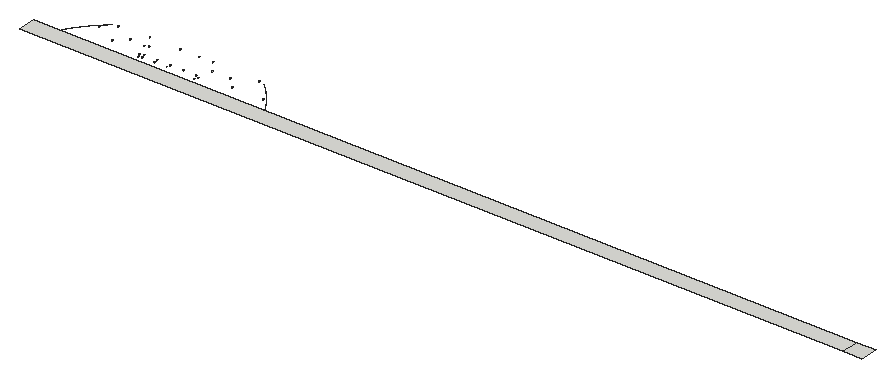
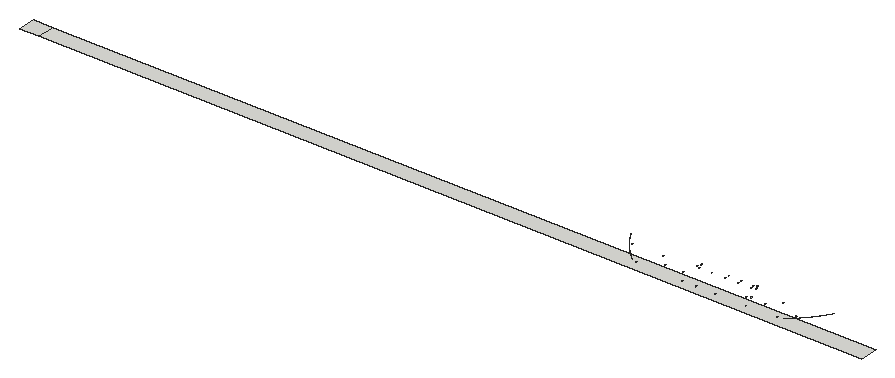
# SketchUp Ruby script. Lengths in inches.
U = 1.inch
M = Sketchup.active_model
def pt(a) = Geom::Point3d.new(a.map { |v| v * U })
def face(e, loops, mat)
  f = e.add_face(loops[0].map { |a| pt(a) })
  loops[1..].each { |l| e.add_face(l.map { |a| pt(a) }).erase! }
  f.material = f.back_material = mat if mat
  f
end
# faces: each face lists its corners as indices into pts; further lists are holes
def faces(e, pts, list, mat = nil) = list.each { |f| face(e, (f[0].is_a?(Array) ? f : [f]).map { |l| l.map { |i| pts[i] } }, mat) }
# xy, xz, yz: faces in a plane at the given z, y or x. An outline is a flat list of corners, or four numbers for a rectangle; further outlines are holes
def ring(l) = l.size == 4 ? [[l[0], l[1]], [l[2], l[1]], [l[2], l[3]], [l[0], l[3]]] : l.each_slice(2).to_a
def flat(e, list, mat, &to3) = list.each { |f| face(e, (f[0].is_a?(Array) ? f : [f]).map { |l| ring(l).map { |u, v| to3.(u, v) } }, mat) }
def xy(e, z, list, mat = nil) = flat(e, list, mat) { |x, y| [x, y, z] }
def xz(e, y, list, mat = nil) = flat(e, list, mat) { |x, z| [x, y, z] }
def yz(e, x, list, mat = nil) = flat(e, list, mat) { |y, z| [x, y, z] }
def lines(e, pts, list) = list.each { |a, b| e.add_line(pt(pts[a]), pt(pts[b])) }
# prism: a flat outline (further loops are holes) pulled along v
def prism(e, loops, v, mat = nil)
  f = face(e, loops, mat); d = Geom::Vector3d.new(v.map { |x| x * U })
  f.pushpull(f.normal.samedirection?(d) ? d.length : -d.length)
end
def box(e, o, s, mat = nil) = prism(e, [[o, [o[0] + s[0], o[1], o[2]], [o[0] + s[0], o[1] + s[1], o[2]], [o[0], o[1] + s[1], o[2]]]], [0, 0, s[2]], mat)
def at(x, y, z, deg = 0) = Geom::Transformation.translation(pt([x, y, z])) * Geom::Transformation.rotation(ORIGIN, Z_AXIS, deg.degrees)
def axes(o, x, y, z) = Geom::Transformation.new([*x, 0, *y, 0, *z, 0, *pt(o).to_a, 1])
def part(name) = M.definitions.add(name)
# library, detail: a bought-in or finely detailed component or shape, given as its bounding box
def library(name, o, s) = part(name).tap { |d| box(d.entities, o, s) }
def detail(e, o, s) = box(e.add_group.entities, o, s)
def put(e, d, t, mat = nil) = e.add_instance(d, t).tap { |i| i.material = mat if mat }
def group(e, t, mat = nil) = e.add_group.tap { |g| g.transformation = t; g.material = mat if mat }.entities
root = M.entities
M.materials.add("[Asphalt_Stamped_Brick]").color = [149, 133, 134]
M.materials.add("[Metal_Steel_Textured_White]").color = [191, 191, 191]
xy(root,0,[[116.615,177.536,303.95,181.5],[303.95,177.536,308.325,181.5]])
xy(root,3.625,[[143.477,177.623,143.471,177.624,143.467,177.626,143.463,177.629,143.459,177.633,143.457,177.638,143.457,177.649,143.459,177.653,143.467,177.661,143.471,177.663,143.482,177.663,143.487,177.661,143.491,177.657,143.494,177.653,143.496,177.649,143.497,177.643,143.496,177.638,143.494,177.633,143.491,177.629,143.487,177.626,143.482,177.624],[156.159,177.623,156.154,177.624,156.149,177.626,156.145,177.629,156.142,177.633,156.14,177.638,156.139,177.643,156.14,177.649,156.142,177.653,156.145,177.657,156.149,177.661,156.154,177.663,156.164,177.663,156.169,177.661,156.173,177.657,156.176,177.653,156.178,177.649,156.179,177.643,156.178,177.638,156.176,177.633,156.173,177.629,156.169,177.626,156.164,177.624],[144.214,177.929,144.209,177.93,144.204,177.932,144.2,177.935,144.197,177.939,144.195,177.944,144.194,177.949,144.195,177.954,144.197,177.959,144.2,177.963,144.204,177.966,144.209,177.968,144.214,177.969,144.219,177.968,144.224,177.966,144.228,177.963,144.232,177.959,144.234,177.954,144.234,177.944,144.232,177.939,144.228,177.935,144.224,177.932,144.219,177.93],[147.016,177.929,147.011,177.93,147.006,177.932,147.002,177.935,146.999,177.939,146.997,177.944,146.996,177.949,146.997,177.954,146.999,177.959,147.002,177.963,147.006,177.966,147.011,177.968,147.016,177.969,147.021,177.968,147.026,177.966,147.03,177.963,147.033,177.959,147.035,177.954,147.036,177.949,147.035,177.944,147.033,177.939,147.03,177.935,147.026,177.932,147.021,177.93],[143.141,178.422,143.136,178.424,143.132,178.428,143.129,178.432,143.127,178.437,143.126,178.442,143.127,178.447,143.129,178.452,143.132,178.456,143.136,178.459,143.141,178.461,143.146,178.462,143.151,178.461,143.156,178.459,143.16,178.456,143.163,178.452,143.165,178.447,143.166,178.442,143.165,178.437,143.163,178.432,143.16,178.428,143.156,178.424,143.151,178.422],
  [156.485,178.422,156.48,178.424,156.476,178.428,156.473,178.432,156.471,178.437,156.47,178.442,156.471,178.447,156.473,178.452,156.476,178.456,156.48,178.459,156.485,178.461,156.49,178.462,156.495,178.461,156.5,178.459,156.504,178.456,156.507,178.452,156.509,178.447,156.51,178.442,156.509,178.437,156.507,178.432,156.504,178.428,156.5,178.424,156.495,178.422],[146.851,178.727,146.846,178.728,146.841,178.73,146.837,178.733,146.833,178.737,146.831,178.742,146.831,178.752,146.833,178.757,146.841,178.765,146.846,178.767,146.856,178.767,146.861,178.765,146.865,178.761,146.868,178.757,146.87,178.752,146.871,178.747,146.87,178.742,146.868,178.737,146.865,178.733,146.861,178.73,146.856,178.728],[155.752,178.727,155.747,178.728,155.742,178.73,155.738,178.733,155.735,178.737,155.733,178.742,155.732,178.747,155.733,178.752,155.735,178.757,155.738,178.761,155.742,178.765,155.747,178.767,155.757,178.767,155.762,178.765,155.766,178.761,155.769,178.757,155.771,178.752,155.772,178.747,155.771,178.742,155.769,178.737,155.766,178.733,155.762,178.73,155.757,178.728],[136.121,179.395,136.116,179.396,136.111,179.398,136.107,179.401,136.104,179.405,136.102,179.41,136.101,179.415,136.102,179.42,136.104,179.425,136.107,179.429,136.111,179.433,136.116,179.435,136.126,179.435,136.131,179.433,136.135,179.429,136.138,179.425,136.14,179.42,136.141,179.415,136.14,179.41,136.138,179.405,136.135,179.401,136.131,179.398,136.126,179.396],[163.515,179.395,163.509,179.396,163.505,179.398,163.501,179.401,163.497,179.405,163.495,179.41,163.495,179.42,163.497,179.425,163.505,179.433,163.509,179.435,163.52,179.435,163.525,179.433,163.529,179.429,163.532,179.425,163.534,179.42,163.535,179.415,163.534,179.41,163.532,179.405,163.529,179.401,163.525,179.398,163.52,179.396],
  [142.641,181.727,142.636,181.728,142.631,181.73,142.627,181.733,142.624,181.737,142.622,181.742,142.621,181.747,142.622,181.752,142.624,181.757,142.627,181.761,142.631,181.765,142.636,181.767,142.646,181.767,142.651,181.765,142.655,181.761,142.658,181.757,142.66,181.752,142.661,181.747,142.66,181.742,142.658,181.737,142.655,181.733,142.651,181.73,142.646,181.728],[156.995,181.727,156.99,181.728,156.985,181.73,156.981,181.733,156.978,181.737,156.976,181.742,156.975,181.747,156.976,181.752,156.978,181.757,156.981,181.761,156.985,181.765,156.99,181.767,157,181.767,157.005,181.765,157.009,181.761,157.012,181.757,157.014,181.752,157.015,181.747,157.014,181.742,157.012,181.737,157.009,181.733,157.005,181.73,157,181.728],[161.174,181.736,161.168,181.737,161.164,181.739,161.159,181.742,161.156,181.746,161.154,181.751,161.154,181.761,161.156,181.766,161.159,181.77,161.164,181.774,161.168,181.776,161.179,181.776,161.184,181.774,161.191,181.766,161.193,181.761,161.194,181.756,161.193,181.751,161.191,181.746,161.1875,181.742,161.184,181.739,161.179,181.737],[133.754,184.074,133.748,184.075,133.744,184.077,133.74,184.08,133.736,184.084,133.734,184.089,133.734,184.099,133.736,184.104,133.74,184.108,133.744,184.111,133.748,184.113,133.754,184.114,133.759,184.113,133.764,184.111,133.768,184.108,133.771,184.104,133.773,184.099,133.774,184.094,133.773,184.089,133.771,184.084,133.768,184.08,133.764,184.077,133.759,184.075],[165.882,184.074,165.877,184.075,165.872,184.077,165.868,184.08,165.865,184.084,165.863,184.089,165.862,184.094,165.863,184.099,165.865,184.104,165.868,184.108,165.872,184.111,165.877,184.113,165.882,184.114,165.887,184.113,165.892,184.111,165.896,184.108,165.899,184.104,165.901,184.099,165.902,184.094,165.901,184.089,165.899,184.084,165.896,184.08,165.892,184.077,165.887,184.075],
  [147.578,184.383,147.572,184.384,147.568,184.386,147.564,184.389,147.56,184.393,147.558,184.398,147.558,184.408,147.56,184.413,147.564,184.417,147.568,184.42,147.572,184.422,147.578,184.423,147.583,184.422,147.588,184.42,147.592,184.417,147.595,184.413,147.597,184.408,147.598,184.403,147.597,184.398,147.595,184.393,147.592,184.389,147.588,184.386,147.583,184.384],[155.076,184.383,155.071,184.384,155.066,184.386,155.0625,184.389,155.059,184.393,155.057,184.398,155.057,184.408,155.059,184.413,155.0625,184.417,155.066,184.42,155.071,184.422,155.076,184.423,155.082,184.422,155.086,184.42,155.091,184.417,155.094,184.413,155.096,184.408,155.096,184.398,155.094,184.393,155.091,184.389,155.086,184.386,155.082,184.384],[140.656,184.422,140.651,184.424,140.643,184.432,140.641,184.437,140.641,184.447,140.643,184.452,140.647,184.456,140.651,184.459,140.656,184.461,140.661,184.462,140.666,184.461,140.671,184.459,140.675,184.456,140.678,184.452,140.68,184.447,140.681,184.442,140.68,184.437,140.678,184.432,140.675,184.428,140.671,184.424,140.666,184.422]],"[Asphalt_Stamped_Brick]")
xy(root,3.625,[[[143.477,177.554,143.454,177.557,143.432,177.566,143.414,177.58,143.4,177.599,143.391,177.62,143.388,177.643,143.391,177.666,143.4,177.688,143.414,177.706,143.432,177.72,143.454,177.729,143.477,177.732,143.5,177.729,143.521,177.72,143.539,177.706,143.554,177.688,143.5625,177.666,143.566,177.643,143.5625,177.62,143.554,177.599,143.539,177.58,143.521,177.566,143.5,177.557],[143.477,177.555,143.499,177.558,143.521,177.567,143.539,177.581,143.553,177.599,143.562,177.621,143.565,177.643,143.562,177.666,143.553,177.6875,143.539,177.706,143.521,177.719,143.499,177.728,143.477,177.731,143.454,177.728,143.433,177.719,143.414,177.706,143.401,177.6875,143.392,177.666,143.389,177.643,143.392,177.621,143.401,177.599,143.414,177.581,143.433,177.567,143.454,177.558]],[[156.159,177.554,156.136,177.557,156.115,177.566,156.096,177.58,156.082,177.599,156.073,177.62,156.07,177.643,156.073,177.666,156.082,177.688,156.096,177.706,156.115,177.72,156.136,177.729,156.159,177.732,156.182,177.729,156.204,177.72,156.222,177.706,156.236,177.688,156.245,177.666,156.248,177.643,156.245,177.62,156.236,177.599,156.222,177.58,156.204,177.566,156.182,177.557],[156.159,177.555,156.182,177.558,156.203,177.567,156.221,177.581,156.235,177.599,156.244,177.621,156.247,177.643,156.244,177.666,156.235,177.6875,156.221,177.706,156.203,177.719,156.182,177.728,156.159,177.731,156.136,177.728,156.115,177.719,156.097,177.706,156.083,177.6875,156.074,177.666,156.071,177.643,156.074,177.621,156.083,177.599,156.097,177.581,156.115,177.567,156.136,177.558]],[[143.477,177.555,143.454,177.558,143.433,177.567,143.414,177.581,143.401,177.599,143.392,177.621,143.389,177.643,143.392,177.666,143.401,177.6875,143.414,177.706,143.433,177.719,143.454,177.728,143.477,177.731,143.499,177.728,143.521,177.719,143.539,177.706,143.553,177.6875,143.562,177.666,143.565,177.643,143.562,177.621,143.553,177.599,143.539,177.581,143.521,177.567,143.499,177.558],[143.477,177.607,143.486,177.608,143.495,177.612,143.503,177.617,143.508,177.625,143.512,177.634,143.513,177.643,143.512,177.653,143.508,177.662,143.503,177.669,143.495,177.675,143.486,177.679,143.477,177.68,143.467,177.679,143.458,177.675,143.451,177.669,143.445,177.662,143.441,177.653,143.44,177.643,143.441,177.634,143.445,177.625,143.451,177.617,143.458,177.612,143.467,177.608]],[[156.159,177.555,156.136,177.558,156.115,177.567,156.097,177.581,156.083,177.599,156.074,177.621,156.071,177.643,156.074,177.666,156.083,177.6875,156.097,177.706,156.115,177.719,156.136,177.728,156.159,177.731,156.182,177.728,156.203,177.719,156.221,177.706,156.235,177.6875,156.244,177.666,156.247,177.643,156.244,177.621,156.235,177.599,156.221,177.581,156.203,177.567,156.182,177.558],[156.159,177.607,156.169,177.608,156.177,177.612,156.185,177.617,156.191,177.625,156.194,177.634,156.196,177.643,156.194,177.653,156.191,177.662,156.185,177.669,156.177,177.675,156.169,177.679,156.159,177.68,156.15,177.679,156.141,177.675,156.133,177.669,156.127,177.662,156.124,177.653,156.123,177.643,156.124,177.634,156.127,177.625,156.133,177.617,156.141,177.612,156.15,177.608]],[[143.477,177.607,143.467,177.608,143.458,177.612,143.451,177.617,143.445,177.625,143.441,177.634,143.44,177.643,143.441,177.653,143.445,177.662,143.451,177.669,143.458,177.675,143.467,177.679,143.477,177.68,143.486,177.679,143.495,177.675,143.503,177.669,143.508,177.662,143.512,177.653,143.513,177.643,143.512,177.634,143.508,177.625,143.503,177.617,143.495,177.612,143.486,177.608],[143.477,177.623,143.482,177.624,143.487,177.626,143.491,177.629,143.494,177.633,143.496,177.638,143.497,177.643,143.496,177.649,143.494,177.653,143.491,177.657,143.487,177.661,143.482,177.663,143.471,177.663,143.467,177.661,143.459,177.653,143.457,177.649,143.457,177.638,143.459,177.633,143.463,177.629,143.467,177.626,143.471,177.624]],
  [[144.214,177.861,144.192,177.864,144.17,177.873,144.152,177.887,144.138,177.905,144.129,177.926,144.126,177.949,144.129,177.972,144.138,177.993,144.152,178.011,144.17,178.025,144.192,178.034,144.214,178.037,144.237,178.034,144.258,178.025,144.276,178.011,144.29,177.993,144.299,177.972,144.302,177.949,144.299,177.926,144.29,177.905,144.276,177.887,144.258,177.873,144.237,177.864],[144.214,177.912,144.224,177.914,144.233,177.917,144.24,177.923,144.246,177.931,144.25,177.939,144.251,177.949,144.25,177.958,144.246,177.967,144.24,177.975,144.233,177.981,144.224,177.984,144.214,177.985,144.205,177.984,144.196,177.981,144.188,177.975,144.183,177.967,144.179,177.958,144.178,177.949,144.179,177.939,144.183,177.931,144.188,177.923,144.196,177.917,144.205,177.914]],[[147.016,177.861,146.993,177.864,146.972,177.873,146.954,177.887,146.94,177.905,146.931,177.926,146.928,177.949,146.931,177.972,146.94,177.993,146.954,178.011,146.972,178.025,146.993,178.034,147.016,178.037,147.039,178.034,147.06,178.025,147.078,178.011,147.092,177.993,147.101,177.972,147.104,177.949,147.101,177.926,147.092,177.905,147.078,177.887,147.06,177.873,147.039,177.864],[147.016,177.912,147.026,177.914,147.034,177.917,147.042,177.923,147.048,177.931,147.051,177.939,147.053,177.949,147.051,177.958,147.048,177.967,147.042,177.975,147.034,177.981,147.026,177.984,147.016,177.985,147.007,177.984,146.998,177.981,146.99,177.975,146.984,177.967,146.981,177.958,146.98,177.949,146.981,177.939,146.984,177.931,146.99,177.923,146.998,177.917,147.007,177.914]],[[144.214,177.912,144.205,177.914,144.196,177.917,144.188,177.923,144.183,177.931,144.179,177.939,144.178,177.949,144.179,177.958,144.183,177.967,144.188,177.975,144.196,177.981,144.205,177.984,144.214,177.985,144.224,177.984,144.233,177.981,144.24,177.975,144.246,177.967,144.25,177.958,144.251,177.949,144.25,177.939,144.246,177.931,144.24,177.923,144.233,177.917,144.224,177.914],[144.214,177.929,144.219,177.93,144.224,177.932,144.228,177.935,144.232,177.939,144.234,177.944,144.234,177.954,144.232,177.959,144.228,177.963,144.224,177.966,144.219,177.968,144.214,177.969,144.209,177.968,144.204,177.966,144.2,177.963,144.197,177.959,144.195,177.954,144.194,177.949,144.195,177.944,144.197,177.939,144.2,177.935,144.204,177.932,144.209,177.93]],[[147.016,177.912,147.007,177.914,146.998,177.917,146.99,177.923,146.984,177.931,146.981,177.939,146.98,177.949,146.981,177.958,146.984,177.967,146.99,177.975,146.998,177.981,147.007,177.984,147.016,177.985,147.026,177.984,147.034,177.981,147.042,177.975,147.048,177.967,147.051,177.958,147.053,177.949,147.051,177.939,147.048,177.931,147.042,177.923,147.034,177.917,147.026,177.914],[147.016,177.929,147.021,177.93,147.026,177.932,147.03,177.935,147.033,177.939,147.035,177.944,147.036,177.949,147.035,177.954,147.033,177.959,147.03,177.963,147.026,177.966,147.021,177.968,147.016,177.969,147.011,177.968,147.006,177.966,147.002,177.963,146.999,177.959,146.997,177.954,146.996,177.949,146.997,177.944,146.999,177.939,147.002,177.935,147.006,177.932,147.011,177.93]],[149.818,177.929,149.813,177.93,149.808,177.932,149.804,177.935,149.801,177.939,149.799,177.944,149.798,177.949,149.799,177.954,149.801,177.959,149.804,177.963,149.808,177.966,149.813,177.968,149.818,177.969],
  [149.818,177.929,149.818,177.969,149.823,177.968,149.828,177.966,149.832,177.963,149.835,177.959,149.837,177.954,149.838,177.949,149.837,177.944,149.835,177.939,149.832,177.935,149.828,177.932,149.823,177.93],[[143.146,178.353,143.123,178.356,143.101,178.365,143.083,178.379,143.069,178.397,143.06,178.419,143.057,178.442,143.06,178.465,143.069,178.486,143.083,178.505,143.101,178.519,143.123,178.528,143.146,178.531,143.169,178.528,143.19,178.519,143.209,178.505,143.223,178.486,143.232,178.465,143.235,178.442,143.232,178.419,143.223,178.397,143.209,178.379,143.19,178.365,143.169,178.356],[143.146,178.354,143.169,178.357,143.19,178.366,143.208,178.38,143.222,178.398,143.231,178.419,143.234,178.442,143.231,178.465,143.222,178.486,143.208,178.504,143.19,178.518,143.169,178.527,143.146,178.53,143.123,178.527,143.102,178.518,143.084,178.504,143.07,178.486,143.061,178.465,143.058,178.442,143.061,178.419,143.07,178.398,143.084,178.38,143.102,178.366,143.123,178.357]],[[143.146,178.354,143.123,178.357,143.102,178.366,143.084,178.38,143.07,178.398,143.061,178.419,143.058,178.442,143.061,178.465,143.07,178.486,143.084,178.504,143.102,178.518,143.123,178.527,143.146,178.53,143.169,178.527,143.19,178.518,143.208,178.504,143.222,178.486,143.231,178.465,143.234,178.442,143.231,178.419,143.222,178.398,143.208,178.38,143.19,178.366,143.169,178.357],[143.146,178.405,143.155,178.406,143.164,178.41,143.172,178.416,143.178,178.423,143.181,178.432,143.183,178.442,143.181,178.451,143.178,178.46,143.172,178.468,143.164,178.473,143.155,178.477,143.146,178.478,143.136,178.477,143.128,178.473,143.12,178.468,143.114,178.46,143.111,178.451,143.109,178.442,143.111,178.432,143.114,178.423,143.12,178.416,143.128,178.41,143.136,178.406]],[[143.146,178.405,143.136,178.406,143.128,178.41,143.12,178.416,143.114,178.423,143.111,178.432,143.109,178.442,143.111,178.451,143.114,178.46,143.12,178.468,143.128,178.473,143.136,178.477,143.146,178.478,143.155,178.477,143.164,178.473,143.172,178.468,143.178,178.46,143.181,178.451,143.183,178.442,143.181,178.432,143.178,178.423,143.172,178.416,143.164,178.41,143.155,178.406],[143.141,178.422,143.151,178.422,143.156,178.424,143.16,178.428,143.163,178.432,143.165,178.437,143.166,178.442,143.165,178.447,143.163,178.452,143.16,178.456,143.156,178.459,143.151,178.461,143.146,178.462,143.141,178.461,143.136,178.459,143.132,178.456,143.129,178.452,143.127,178.447,143.126,178.442,143.127,178.437,143.129,178.432,143.132,178.428,143.136,178.424]],[[156.49,178.405,156.48,178.406,156.472,178.41,156.464,178.416,156.458,178.423,156.455,178.432,156.453,178.442,156.455,178.451,156.458,178.46,156.464,178.468,156.472,178.473,156.48,178.477,156.49,178.478,156.499,178.477,156.508,178.473,156.516,178.468,156.522,178.46,156.525,178.451,156.526,178.442,156.525,178.432,156.522,178.423,156.516,178.416,156.508,178.41,156.499,178.406],[156.485,178.422,156.495,178.422,156.5,178.424,156.504,178.428,156.507,178.432,156.509,178.437,156.51,178.442,156.509,178.447,156.507,178.452,156.504,178.456,156.5,178.459,156.495,178.461,156.49,178.462,156.485,178.461,156.48,178.459,156.476,178.456,156.473,178.452,156.471,178.447,156.47,178.442,156.471,178.437,156.473,178.432,156.476,178.428,156.48,178.424]],
  [[143.884,178.658,143.861,178.661,143.839,178.67,143.821,178.684,143.807,178.703,143.798,178.724,143.795,178.747,143.798,178.77,143.807,178.792,143.821,178.81,143.839,178.824,143.861,178.833,143.884,178.836,143.907,178.833,143.928,178.824,143.946,178.81,143.961,178.792,143.969,178.77,143.972,178.747,143.969,178.724,143.961,178.703,143.946,178.684,143.928,178.67,143.907,178.661],[143.884,178.659,143.906,178.662,143.928,178.671,143.946,178.685,143.96,178.703,143.969,178.725,143.972,178.747,143.969,178.77,143.96,178.791,143.946,178.809,143.928,178.823,143.906,178.832,143.884,178.835,143.861,178.832,143.84,178.823,143.821,178.809,143.807,178.791,143.799,178.77,143.796,178.747,143.799,178.725,143.807,178.703,143.821,178.685,143.84,178.671,143.861,178.662]],[[146.851,178.658,146.828,178.661,146.806,178.67,146.788,178.684,146.774,178.703,146.765,178.724,146.762,178.747,146.765,178.77,146.774,178.792,146.788,178.81,146.806,178.824,146.828,178.833,146.851,178.836,146.874,178.833,146.895,178.824,146.914,178.81,146.928,178.792,146.937,178.77,146.94,178.747,146.937,178.724,146.928,178.703,146.914,178.684,146.895,178.67,146.874,178.661],[146.851,178.659,146.873,178.662,146.895,178.671,146.913,178.685,146.927,178.703,146.936,178.725,146.939,178.747,146.936,178.77,146.927,178.791,146.913,178.809,146.895,178.823,146.873,178.832,146.851,178.835,146.828,178.832,146.807,178.823,146.789,178.809,146.775,178.791,146.766,178.77,146.763,178.747,146.766,178.725,146.775,178.703,146.789,178.685,146.807,178.671,146.828,178.662]],[149.818,178.658,149.795,178.661,149.773,178.67,149.755,178.684,149.741,178.703,149.732,178.724,149.729,178.747,149.732,178.77,149.741,178.792,149.755,178.81,149.773,178.824,149.795,178.833,149.818,178.836,149.818,178.835,149.795,178.832,149.774,178.823,149.756,178.809,149.742,178.791,149.733,178.77,149.73,178.747,149.733,178.725,149.742,178.703,149.756,178.685,149.774,178.671,149.795,178.662,149.818,178.659],[149.818,178.658,149.818,178.659,149.841,178.662,149.862,178.671,149.88,178.685,149.894,178.703,149.903,178.725,149.906,178.747,149.903,178.77,149.894,178.791,149.88,178.809,149.862,178.823,149.841,178.832,149.818,178.835,149.818,178.836,149.841,178.833,149.862,178.824,149.881,178.81,149.895,178.792,149.904,178.77,149.907,178.747,149.904,178.724,149.895,178.703,149.881,178.684,149.862,178.67,149.841,178.661],[[146.851,178.659,146.828,178.662,146.807,178.671,146.789,178.685,146.775,178.703,146.766,178.725,146.763,178.747,146.766,178.77,146.775,178.791,146.789,178.809,146.807,178.823,146.828,178.832,146.851,178.835,146.873,178.832,146.895,178.823,146.913,178.809,146.927,178.791,146.936,178.77,146.939,178.747,146.936,178.725,146.927,178.703,146.913,178.685,146.895,178.671,146.873,178.662],[146.851,178.711,146.86,178.712,146.869,178.716,146.877,178.721,146.882,178.729,146.886,178.738,146.887,178.747,146.886,178.757,146.882,178.766,146.877,178.773,146.869,178.779,146.86,178.783,146.851,178.784,146.841,178.783,146.832,178.779,146.825,178.773,146.819,178.766,146.815,178.757,146.814,178.747,146.815,178.738,146.819,178.729,146.825,178.721,146.832,178.716,146.841,178.712]],
  [[152.785,178.659,152.762,178.662,152.741,178.671,152.723,178.685,152.709,178.703,152.7,178.725,152.697,178.747,152.7,178.77,152.709,178.791,152.723,178.809,152.741,178.823,152.762,178.832,152.785,178.835,152.808,178.832,152.829,178.823,152.847,178.809,152.861,178.791,152.87,178.77,152.873,178.747,152.87,178.725,152.861,178.703,152.847,178.685,152.829,178.671,152.808,178.662],[152.785,178.711,152.795,178.712,152.803,178.716,152.811,178.721,152.817,178.729,152.82,178.738,152.822,178.747,152.82,178.757,152.817,178.766,152.811,178.773,152.803,178.779,152.795,178.783,152.785,178.784,152.776,178.783,152.767,178.779,152.759,178.773,152.753,178.766,152.75,178.757,152.748,178.747,152.75,178.738,152.753,178.729,152.759,178.721,152.767,178.716,152.776,178.712]],[[155.752,178.659,155.729,178.662,155.708,178.671,155.69,178.685,155.676,178.703,155.667,178.725,155.664,178.747,155.667,178.77,155.676,178.791,155.69,178.809,155.708,178.823,155.729,178.832,155.752,178.835,155.775,178.832,155.796,178.823,155.814,178.809,155.828,178.791,155.837,178.77,155.84,178.747,155.837,178.725,155.828,178.703,155.814,178.685,155.796,178.671,155.775,178.662],[155.752,178.711,155.762,178.712,155.771,178.716,155.778,178.721,155.784,178.729,155.788,178.738,155.789,178.747,155.788,178.757,155.784,178.766,155.778,178.773,155.771,178.779,155.762,178.783,155.752,178.784,155.743,178.783,155.734,178.779,155.726,178.773,155.721,178.766,155.717,178.757,155.716,178.747,155.717,178.738,155.721,178.729,155.726,178.721,155.734,178.716,155.743,178.712]],[[146.851,178.711,146.841,178.712,146.832,178.716,146.825,178.721,146.819,178.729,146.815,178.738,146.814,178.747,146.815,178.757,146.819,178.766,146.825,178.773,146.832,178.779,146.841,178.783,146.851,178.784,146.86,178.783,146.869,178.779,146.877,178.773,146.882,178.766,146.886,178.757,146.887,178.747,146.886,178.738,146.882,178.729,146.877,178.721,146.869,178.716,146.86,178.712],[146.851,178.727,146.856,178.728,146.861,178.73,146.865,178.733,146.868,178.737,146.87,178.742,146.871,178.747,146.87,178.752,146.868,178.757,146.865,178.761,146.861,178.765,146.856,178.767,146.846,178.767,146.841,178.765,146.833,178.757,146.831,178.752,146.831,178.742,146.833,178.737,146.837,178.733,146.841,178.73,146.846,178.728]],[149.818,178.711,149.818,178.727,149.823,178.728,149.828,178.73,149.832,178.733,149.835,178.737,149.837,178.742,149.838,178.747,149.837,178.752,149.835,178.757,149.832,178.761,149.828,178.765,149.823,178.767,149.818,178.767,149.818,178.784,149.827,178.783,149.836,178.779,149.844,178.773,149.85,178.766,149.853,178.757,149.854,178.747,149.853,178.738,149.85,178.729,149.844,178.721,149.836,178.716,149.827,178.712],[[155.752,178.711,155.743,178.712,155.734,178.716,155.726,178.721,155.721,178.729,155.717,178.738,155.716,178.747,155.717,178.757,155.721,178.766,155.726,178.773,155.734,178.779,155.743,178.783,155.752,178.784,155.762,178.783,155.771,178.779,155.778,178.773,155.784,178.766,155.788,178.757,155.789,178.747,155.788,178.738,155.784,178.729,155.778,178.721,155.771,178.716,155.762,178.712],[155.752,178.727,155.757,178.728,155.762,178.73,155.766,178.733,155.769,178.737,155.771,178.742,155.772,178.747,155.771,178.752,155.769,178.757,155.766,178.761,155.762,178.765,155.757,178.767,155.747,178.767,155.742,178.765,155.738,178.761,155.735,178.757,155.733,178.752,155.732,178.747,155.733,178.742,155.735,178.737,155.738,178.733,155.742,178.73,155.747,178.728]],
  [[136.121,179.326,136.098,179.329,136.077,179.338,136.058,179.352,136.044,179.371,136.035,179.392,136.032,179.415,136.035,179.438,136.044,179.46,136.058,179.478,136.077,179.492,136.098,179.501,136.121,179.504,136.144,179.501,136.166,179.492,136.184,179.478,136.198,179.46,136.207,179.438,136.21,179.415,136.207,179.392,136.198,179.371,136.184,179.352,136.166,179.338,136.144,179.329],[136.121,179.327,136.144,179.33,136.165,179.339,136.183,179.353,136.197,179.371,136.206,179.392,136.209,179.415,136.206,179.438,136.197,179.459,136.183,179.477,136.165,179.491,136.144,179.5,136.121,179.503,136.098,179.5,136.077,179.491,136.059,179.477,136.045,179.459,136.036,179.438,136.033,179.415,136.036,179.392,136.045,179.371,136.059,179.353,136.077,179.339,136.098,179.33]],[[163.515,179.326,163.492,179.329,163.47,179.338,163.452,179.352,163.4375,179.371,163.429,179.392,163.426,179.415,163.429,179.438,163.4375,179.46,163.452,179.478,163.47,179.492,163.492,179.501,163.515,179.504,163.538,179.501,163.559,179.492,163.577,179.478,163.592,179.46,163.6,179.438,163.604,179.415,163.6,179.392,163.592,179.371,163.577,179.352,163.559,179.338,163.538,179.329],[163.515,179.327,163.537,179.33,163.559,179.339,163.577,179.353,163.591,179.371,163.6,179.392,163.603,179.415,163.6,179.438,163.591,179.459,163.577,179.477,163.559,179.491,163.537,179.5,163.515,179.503,163.492,179.5,163.471,179.491,163.452,179.477,163.438,179.459,163.43,179.438,163.427,179.415,163.43,179.392,163.438,179.371,163.452,179.353,163.471,179.339,163.492,179.33]],[[136.121,179.327,136.098,179.33,136.077,179.339,136.059,179.353,136.045,179.371,136.036,179.392,136.033,179.415,136.036,179.438,136.045,179.459,136.059,179.477,136.077,179.491,136.098,179.5,136.121,179.503,136.144,179.5,136.165,179.491,136.183,179.477,136.197,179.459,136.206,179.438,136.209,179.415,136.206,179.392,136.197,179.371,136.183,179.353,136.165,179.339,136.144,179.33],[136.121,179.379,136.131,179.38,136.139,179.384,136.147,179.389,136.153,179.397,136.157,179.406,136.158,179.415,136.157,179.425,136.153,179.434,136.147,179.441,136.139,179.447,136.131,179.451,136.121,179.452,136.112,179.451,136.103,179.447,136.095,179.441,136.089,179.434,136.086,179.425,136.085,179.415,136.086,179.406,136.089,179.397,136.095,179.389,136.103,179.384,136.112,179.38]],[[170.535,179.354,170.512,179.357,170.491,179.366,170.472,179.38,170.458,179.398,170.45,179.419,170.447,179.442,170.45,179.464,170.458,179.486,170.472,179.504,170.491,179.518,170.512,179.527,170.535,179.53,170.557,179.527,170.579,179.518,170.597,179.504,170.611,179.486,170.62,179.464,170.623,179.442,170.62,179.419,170.611,179.398,170.597,179.38,170.579,179.366,170.557,179.357],[170.535,179.405,170.544,179.406,170.553,179.41,170.561,179.416,170.566,179.423,170.57,179.432,170.571,179.442,170.57,179.451,170.566,179.46,170.561,179.468,170.553,179.473,170.544,179.477,170.535,179.478,170.525,179.477,170.516,179.473,170.509,179.468,170.503,179.46,170.499,179.451,170.498,179.442,170.499,179.432,170.503,179.423,170.509,179.416,170.516,179.41,170.525,179.406]],[[136.121,179.379,136.112,179.38,136.103,179.384,136.095,179.389,136.089,179.397,136.086,179.406,136.085,179.415,136.086,179.425,136.089,179.434,136.095,179.441,136.103,179.447,136.112,179.451,136.121,179.452,136.131,179.451,136.139,179.447,136.147,179.441,136.153,179.434,136.157,179.425,136.158,179.415,136.157,179.406,136.153,179.397,136.147,179.389,136.139,179.384,136.131,179.38],[136.121,179.395,136.126,179.396,136.131,179.398,136.135,179.401,136.138,179.405,136.14,179.41,136.141,179.415,136.14,179.42,136.138,179.425,136.135,179.429,136.131,179.433,136.126,179.435,136.116,179.435,136.111,179.433,136.107,179.429,136.104,179.425,136.102,179.42,136.101,179.415,136.102,179.41,136.104,179.405,136.107,179.401,136.111,179.398,136.116,179.396]],
  [[163.515,179.379,163.505,179.38,163.496,179.384,163.489,179.389,163.483,179.397,163.479,179.406,163.478,179.415,163.479,179.425,163.483,179.434,163.489,179.441,163.496,179.447,163.505,179.451,163.515,179.452,163.524,179.451,163.533,179.447,163.541,179.441,163.546,179.434,163.55,179.425,163.551,179.415,163.55,179.406,163.546,179.397,163.541,179.389,163.533,179.384,163.524,179.38],[163.515,179.395,163.52,179.396,163.525,179.398,163.529,179.401,163.532,179.405,163.534,179.41,163.535,179.415,163.534,179.42,163.532,179.425,163.529,179.429,163.525,179.433,163.52,179.435,163.509,179.435,163.505,179.433,163.497,179.425,163.495,179.42,163.495,179.41,163.497,179.405,163.501,179.401,163.505,179.398,163.509,179.396]],[170.529,179.422,170.525,179.424,170.517,179.432,170.515,179.437,170.515,179.447,170.517,179.452,170.521,179.456,170.525,179.459,170.529,179.461,170.535,179.462,170.54,179.461,170.545,179.459,170.549,179.456,170.552,179.452,170.554,179.447,170.555,179.442,170.554,179.437,170.552,179.432,170.549,179.428,170.545,179.424,170.54,179.422],[[141.903,181.353,141.88,181.356,141.859,181.365,141.84,181.379,141.826,181.397,141.817,181.419,141.814,181.442,141.817,181.465,141.826,181.486,141.84,181.505,141.859,181.519,141.88,181.528,141.903,181.531,141.926,181.528,141.948,181.519,141.966,181.505,141.98,181.486,141.989,181.465,141.992,181.442,141.989,181.419,141.98,181.397,141.966,181.379,141.948,181.365,141.926,181.356],[141.903,181.354,141.926,181.357,141.947,181.366,141.965,181.38,141.979,181.398,141.988,181.419,141.991,181.442,141.988,181.464,141.979,181.486,141.965,181.504,141.947,181.518,141.926,181.527,141.903,181.53,141.881,181.527,141.859,181.518,141.841,181.504,141.827,181.486,141.818,181.464,141.815,181.442,141.818,181.419,141.827,181.398,141.841,181.38,141.859,181.366,141.881,181.357]],[[142.641,181.658,142.618,181.661,142.597,181.67,142.578,181.684,142.564,181.703,142.555,181.724,142.552,181.747,142.555,181.77,142.564,181.792,142.578,181.81,142.597,181.824,142.618,181.833,142.641,181.836,142.664,181.833,142.685,181.824,142.704,181.81,142.718,181.792,142.727,181.77,142.73,181.747,142.727,181.724,142.718,181.703,142.704,181.684,142.685,181.67,142.664,181.661],[142.641,181.659,142.664,181.662,142.685,181.671,142.703,181.685,142.717,181.703,142.726,181.725,142.729,181.747,142.726,181.77,142.717,181.791,142.703,181.809,142.685,181.823,142.664,181.832,142.641,181.835,142.618,181.832,142.597,181.823,142.579,181.809,142.565,181.791,142.556,181.77,142.553,181.747,142.556,181.725,142.565,181.703,142.579,181.685,142.597,181.671,142.618,181.662]],[[142.641,181.659,142.618,181.662,142.597,181.671,142.579,181.685,142.565,181.703,142.556,181.725,142.553,181.747,142.556,181.77,142.565,181.791,142.579,181.809,142.597,181.823,142.618,181.832,142.641,181.835,142.664,181.832,142.685,181.823,142.703,181.809,142.717,181.791,142.726,181.77,142.729,181.747,142.726,181.725,142.717,181.703,142.703,181.685,142.685,181.671,142.664,181.662],[142.641,181.711,142.65,181.712,142.659,181.716,142.667,181.721,142.673,181.729,142.676,181.738,142.678,181.747,142.676,181.757,142.673,181.766,142.667,181.773,142.659,181.779,142.65,181.783,142.641,181.784,142.631,181.783,142.623,181.779,142.615,181.773,142.609,181.766,142.606,181.757,142.604,181.747,142.606,181.738,142.609,181.729,142.615,181.721,142.623,181.716,142.631,181.712]],
  [[156.995,181.659,156.972,181.662,156.951,181.671,156.933,181.685,156.919,181.703,156.91,181.725,156.907,181.747,156.91,181.77,156.919,181.791,156.933,181.809,156.951,181.823,156.972,181.832,156.995,181.835,157.018,181.832,157.039,181.823,157.057,181.809,157.071,181.791,157.08,181.77,157.083,181.747,157.08,181.725,157.071,181.703,157.057,181.685,157.039,181.671,157.018,181.662],[156.995,181.711,157.004,181.712,157.013,181.716,157.021,181.721,157.027,181.729,157.03,181.738,157.031,181.747,157.03,181.757,157.027,181.766,157.021,181.773,157.013,181.779,157.004,181.783,156.995,181.784,156.985,181.783,156.977,181.779,156.969,181.773,156.963,181.766,156.959,181.757,156.958,181.747,156.959,181.738,156.963,181.729,156.969,181.721,156.977,181.716,156.985,181.712]],[[138.462,181.667,138.439,181.67,138.418,181.679,138.399,181.693,138.385,181.712,138.376,181.733,138.373,181.756,138.376,181.779,138.385,181.801,138.399,181.819,138.418,181.833,138.439,181.842,138.462,181.845,138.485,181.842,138.507,181.833,138.525,181.819,138.539,181.801,138.548,181.779,138.551,181.756,138.548,181.733,138.539,181.712,138.525,181.693,138.507,181.679,138.485,181.67],[138.462,181.668,138.485,181.671,138.506,181.68,138.524,181.694,138.538,181.712,138.547,181.734,138.55,181.756,138.547,181.779,138.538,181.8,138.524,181.818,138.506,181.832,138.485,181.841,138.462,181.844,138.439,181.841,138.418,181.832,138.4,181.818,138.386,181.8,138.377,181.779,138.374,181.756,138.377,181.734,138.386,181.712,138.4,181.694,138.418,181.68,138.439,181.671]],[[161.174,181.667,161.151,181.67,161.129,181.679,161.111,181.693,161.097,181.712,161.088,181.733,161.085,181.756,161.088,181.779,161.097,181.801,161.111,181.819,161.129,181.833,161.151,181.842,161.174,181.845,161.197,181.842,161.218,181.833,161.236,181.819,161.251,181.801,161.259,181.779,161.262,181.756,161.259,181.733,161.251,181.712,161.236,181.693,161.218,181.679,161.197,181.67],[161.174,181.668,161.196,181.671,161.218,181.68,161.236,181.694,161.25,181.712,161.258,181.734,161.261,181.756,161.258,181.779,161.25,181.8,161.236,181.818,161.218,181.832,161.196,181.841,161.174,181.844,161.151,181.841,161.13,181.832,161.111,181.818,161.097,181.8,161.089,181.779,161.086,181.756,161.089,181.734,161.097,181.712,161.111,181.694,161.13,181.68,161.151,181.671]],[[138.462,181.668,138.439,181.671,138.418,181.68,138.4,181.694,138.386,181.712,138.377,181.734,138.374,181.756,138.377,181.779,138.386,181.8,138.4,181.818,138.418,181.832,138.439,181.841,138.462,181.844,138.485,181.841,138.506,181.832,138.524,181.818,138.538,181.8,138.547,181.779,138.55,181.756,138.547,181.734,138.538,181.712,138.524,181.694,138.506,181.68,138.485,181.671],[138.462,181.72,138.472,181.721,138.481,181.725,138.488,181.73,138.494,181.738,138.498,181.747,138.499,181.756,138.498,181.766,138.494,181.775,138.488,181.782,138.481,181.788,138.472,181.792,138.462,181.793,138.453,181.792,138.444,181.788,138.436,181.782,138.431,181.775,138.427,181.766,138.426,181.756,138.427,181.747,138.431,181.738,138.436,181.73,138.444,181.725,138.453,181.721]],[[142.641,181.711,142.631,181.712,142.623,181.716,142.615,181.721,142.609,181.729,142.606,181.738,142.604,181.747,142.606,181.757,142.609,181.766,142.615,181.773,142.623,181.779,142.631,181.783,142.641,181.784,142.65,181.783,142.659,181.779,142.667,181.773,142.673,181.766,142.676,181.757,142.678,181.747,142.676,181.738,142.673,181.729,142.667,181.721,142.659,181.716,142.65,181.712],[142.641,181.727,142.646,181.728,142.651,181.73,142.655,181.733,142.658,181.737,142.66,181.742,142.661,181.747,142.66,181.752,142.658,181.757,142.655,181.761,142.651,181.765,142.646,181.767,142.636,181.767,142.631,181.765,142.627,181.761,142.624,181.757,142.622,181.752,142.621,181.747,142.622,181.742,142.624,181.737,142.627,181.733,142.631,181.73,142.636,181.728]],
  [[156.995,181.711,156.985,181.712,156.977,181.716,156.969,181.721,156.963,181.729,156.959,181.738,156.958,181.747,156.959,181.757,156.963,181.766,156.969,181.773,156.977,181.779,156.985,181.783,156.995,181.784,157.004,181.783,157.013,181.779,157.021,181.773,157.027,181.766,157.03,181.757,157.031,181.747,157.03,181.738,157.027,181.729,157.021,181.721,157.013,181.716,157.004,181.712],[156.995,181.727,157,181.728,157.005,181.73,157.009,181.733,157.012,181.737,157.014,181.742,157.015,181.747,157.014,181.752,157.012,181.757,157.009,181.761,157.005,181.765,157,181.767,156.99,181.767,156.985,181.765,156.981,181.761,156.978,181.757,156.976,181.752,156.975,181.747,156.976,181.742,156.978,181.737,156.981,181.733,156.985,181.73,156.99,181.728]],[[161.174,181.72,161.164,181.721,161.155,181.725,161.148,181.73,161.142,181.738,161.138,181.747,161.137,181.756,161.138,181.766,161.142,181.775,161.148,181.782,161.155,181.788,161.164,181.792,161.174,181.793,161.183,181.792,161.192,181.788,161.199,181.782,161.205,181.775,161.209,181.766,161.21,181.756,161.209,181.747,161.205,181.738,161.199,181.73,161.192,181.725,161.183,181.721],[161.174,181.736,161.179,181.737,161.184,181.739,161.1875,181.742,161.191,181.746,161.193,181.751,161.194,181.756,161.193,181.761,161.191,181.766,161.184,181.774,161.179,181.776,161.168,181.776,161.164,181.774,161.159,181.77,161.156,181.766,161.154,181.761,161.154,181.751,161.156,181.746,161.159,181.742,161.164,181.739,161.168,181.737]],[[131.281,181.826,131.258,181.829,131.236,181.837,131.218,181.852,131.204,181.87,131.195,181.891,131.192,181.914,131.195,181.9375,131.204,181.959,131.218,181.977,131.236,181.991,131.258,182,131.281,182.003,131.304,182,131.325,181.991,131.344,181.977,131.358,181.959,131.367,181.9375,131.37,181.914,131.367,181.891,131.358,181.87,131.344,181.852,131.325,181.837,131.304,181.829],[131.281,181.827,131.304,181.83,131.325,181.838,131.343,181.852,131.357,181.87,131.366,181.892,131.369,181.914,131.366,181.937,131.357,181.958,131.343,181.977,131.325,181.991,131.304,181.999,131.281,182.002,131.258,181.999,131.237,181.991,131.219,181.977,131.205,181.958,131.196,181.937,131.193,181.914,131.196,181.892,131.205,181.87,131.219,181.852,131.237,181.838,131.258,181.83]],[[131.281,181.827,131.258,181.83,131.237,181.838,131.219,181.852,131.205,181.87,131.196,181.892,131.193,181.914,131.196,181.937,131.205,181.958,131.219,181.977,131.237,181.991,131.258,181.999,131.281,182.002,131.304,181.999,131.325,181.991,131.343,181.977,131.357,181.958,131.366,181.937,131.369,181.914,131.366,181.892,131.357,181.87,131.343,181.852,131.325,181.838,131.304,181.83],[131.281,181.878,131.29,181.879,131.299,181.883,131.307,181.889,131.3125,181.896,131.316,181.905,131.317,181.914,131.316,181.924,131.3125,181.933,131.307,181.94,131.299,181.946,131.29,181.95,131.281,181.951,131.271,181.95,131.263,181.946,131.255,181.94,131.249,181.933,131.246,181.924,131.244,181.914,131.246,181.905,131.249,181.896,131.255,181.889,131.263,181.883,131.271,181.879]],[[133.754,184.005,133.731,184.008,133.709,184.017,133.691,184.031,133.677,184.05,133.668,184.071,133.665,184.094,133.668,184.117,133.677,184.139,133.691,184.157,133.709,184.171,133.731,184.18,133.754,184.183,133.777,184.18,133.798,184.171,133.816,184.157,133.831,184.139,133.839,184.117,133.843,184.094,133.839,184.071,133.831,184.05,133.816,184.031,133.798,184.017,133.777,184.008],[133.754,184.006,133.776,184.009,133.798,184.018,133.816,184.032,133.83,184.05,133.839,184.071,133.842,184.094,133.839,184.117,133.83,184.138,133.816,184.156,133.798,184.17,133.776,184.179,133.754,184.182,133.731,184.179,133.71,184.17,133.691,184.156,133.677,184.138,133.669,184.117,133.666,184.094,133.669,184.071,133.677,184.05,133.691,184.032,133.71,184.018,133.731,184.009]],
  [[165.882,184.005,165.859,184.008,165.838,184.017,165.819,184.031,165.805,184.05,165.796,184.071,165.793,184.094,165.796,184.117,165.805,184.139,165.819,184.157,165.838,184.171,165.859,184.18,165.882,184.183,165.905,184.18,165.927,184.171,165.945,184.157,165.959,184.139,165.968,184.117,165.971,184.094,165.968,184.071,165.959,184.05,165.945,184.031,165.927,184.017,165.905,184.008],[165.882,184.006,165.905,184.009,165.926,184.018,165.944,184.032,165.958,184.05,165.967,184.071,165.97,184.094,165.967,184.117,165.958,184.138,165.944,184.156,165.926,184.17,165.905,184.179,165.882,184.182,165.859,184.179,165.838,184.17,165.82,184.156,165.806,184.138,165.797,184.117,165.794,184.094,165.797,184.071,165.806,184.05,165.82,184.032,165.838,184.018,165.859,184.009]],[[165.882,184.006,165.859,184.009,165.838,184.018,165.82,184.032,165.806,184.05,165.797,184.071,165.794,184.094,165.797,184.117,165.806,184.138,165.82,184.156,165.838,184.17,165.859,184.179,165.882,184.182,165.905,184.179,165.926,184.17,165.944,184.156,165.958,184.138,165.967,184.117,165.97,184.094,165.967,184.071,165.958,184.05,165.944,184.032,165.926,184.018,165.905,184.009],[165.882,184.058,165.892,184.059,165.9,184.0625,165.908,184.068,165.914,184.076,165.917,184.085,165.919,184.094,165.917,184.104,165.914,184.112,165.908,184.12,165.9,184.126,165.892,184.13,165.882,184.131,165.873,184.13,165.864,184.126,165.856,184.12,165.85,184.112,165.847,184.104,165.846,184.094,165.847,184.085,165.85,184.076,165.856,184.068,165.864,184.0625,165.873,184.059]],[[133.754,184.058,133.744,184.059,133.735,184.0625,133.728,184.068,133.722,184.076,133.718,184.085,133.717,184.094,133.718,184.104,133.722,184.112,133.728,184.12,133.735,184.126,133.744,184.13,133.754,184.131,133.763,184.13,133.772,184.126,133.78,184.12,133.785,184.112,133.789,184.104,133.79,184.094,133.789,184.085,133.785,184.076,133.78,184.068,133.772,184.0625,133.763,184.059],[133.754,184.074,133.759,184.075,133.764,184.077,133.768,184.08,133.771,184.084,133.773,184.089,133.774,184.094,133.773,184.099,133.771,184.104,133.768,184.108,133.764,184.111,133.759,184.113,133.754,184.114,133.748,184.113,133.744,184.111,133.74,184.108,133.736,184.104,133.734,184.099,133.734,184.089,133.736,184.084,133.74,184.08,133.744,184.077,133.748,184.075]],[[165.882,184.058,165.873,184.059,165.864,184.0625,165.856,184.068,165.85,184.076,165.847,184.085,165.846,184.094,165.847,184.104,165.85,184.112,165.856,184.12,165.864,184.126,165.873,184.13,165.882,184.131,165.892,184.13,165.9,184.126,165.908,184.12,165.914,184.112,165.917,184.104,165.919,184.094,165.917,184.085,165.914,184.076,165.908,184.068,165.9,184.0625,165.892,184.059],[165.882,184.074,165.887,184.075,165.892,184.077,165.896,184.08,165.899,184.084,165.901,184.089,165.902,184.094,165.901,184.099,165.899,184.104,165.896,184.108,165.892,184.111,165.887,184.113,165.882,184.114,165.877,184.113,165.872,184.111,165.868,184.108,165.865,184.104,165.863,184.099,165.862,184.094,165.863,184.089,165.865,184.084,165.868,184.08,165.872,184.077,165.877,184.075]],[[147.578,184.314,147.555,184.317,147.533,184.326,147.515,184.34,147.501,184.358,147.492,184.38,147.489,184.403,147.492,184.426,147.501,184.447,147.515,184.466,147.533,184.48,147.555,184.489,147.578,184.492,147.601,184.489,147.622,184.48,147.641,184.466,147.655,184.447,147.664,184.426,147.667,184.403,147.664,184.38,147.655,184.358,147.641,184.34,147.622,184.326,147.601,184.317],[147.578,184.315,147.6,184.318,147.622,184.327,147.64,184.341,147.654,184.359,147.663,184.38,147.666,184.403,147.663,184.426,147.654,184.447,147.64,184.465,147.622,184.479,147.6,184.488,147.578,184.491,147.555,184.488,147.534,184.479,147.515,184.465,147.502,184.447,147.493,184.426,147.49,184.403,147.493,184.38,147.502,184.359,147.515,184.341,147.534,184.327,147.555,184.318]],
  [[152.058,184.314,152.035,184.317,152.014,184.326,151.995,184.34,151.981,184.358,151.972,184.38,151.969,184.403,151.972,184.426,151.981,184.447,151.995,184.466,152.014,184.48,152.035,184.489,152.058,184.492,152.081,184.489,152.103,184.48,152.121,184.466,152.135,184.447,152.144,184.426,152.147,184.403,152.144,184.38,152.135,184.358,152.121,184.34,152.103,184.326,152.081,184.317],[152.058,184.315,152.081,184.318,152.102,184.327,152.12,184.341,152.134,184.359,152.143,184.38,152.146,184.403,152.143,184.426,152.134,184.447,152.12,184.465,152.102,184.479,152.081,184.488,152.058,184.491,152.035,184.488,152.014,184.479,151.996,184.465,151.982,184.447,151.973,184.426,151.97,184.403,151.973,184.38,151.982,184.359,151.996,184.341,152.014,184.327,152.035,184.318]],[[147.578,184.315,147.555,184.318,147.534,184.327,147.515,184.341,147.502,184.359,147.493,184.38,147.49,184.403,147.493,184.426,147.502,184.447,147.515,184.465,147.534,184.479,147.555,184.488,147.578,184.491,147.6,184.488,147.622,184.479,147.64,184.465,147.654,184.447,147.663,184.426,147.666,184.403,147.663,184.38,147.654,184.359,147.64,184.341,147.622,184.327,147.6,184.318],[147.578,184.366,147.587,184.368,147.596,184.371,147.604,184.377,147.609,184.385,147.613,184.393,147.614,184.403,147.613,184.412,147.609,184.421,147.604,184.429,147.596,184.435,147.587,184.438,147.578,184.44,147.568,184.438,147.559,184.435,147.552,184.429,147.546,184.421,147.542,184.412,147.541,184.403,147.542,184.393,147.546,184.385,147.552,184.377,147.559,184.371,147.568,184.368]],[[152.058,184.315,152.035,184.318,152.014,184.327,151.996,184.341,151.982,184.359,151.973,184.38,151.97,184.403,151.973,184.426,151.982,184.447,151.996,184.465,152.014,184.479,152.035,184.488,152.058,184.491,152.081,184.488,152.102,184.479,152.12,184.465,152.134,184.447,152.143,184.426,152.146,184.403,152.143,184.38,152.134,184.359,152.12,184.341,152.102,184.327,152.081,184.318],[152.058,184.366,152.068,184.368,152.076,184.371,152.084,184.377,152.09,184.385,152.093,184.393,152.095,184.403,152.093,184.412,152.09,184.421,152.084,184.429,152.076,184.435,152.068,184.438,152.058,184.44,152.049,184.438,152.04,184.435,152.032,184.429,152.026,184.421,152.023,184.412,152.022,184.403,152.023,184.393,152.026,184.385,152.032,184.377,152.04,184.371,152.049,184.368]],[[155.076,184.315,155.054,184.318,155.033,184.327,155.014,184.341,155,184.359,154.992,184.38,154.989,184.403,154.992,184.426,155,184.447,155.014,184.465,155.033,184.479,155.054,184.488,155.076,184.491,155.099,184.488,155.12,184.479,155.139,184.465,155.153,184.447,155.161,184.426,155.164,184.403,155.161,184.38,155.153,184.359,155.139,184.341,155.12,184.327,155.099,184.318],[155.076,184.366,155.086,184.368,155.095,184.371,155.102,184.377,155.108,184.385,155.112,184.393,155.113,184.403,155.112,184.412,155.108,184.421,155.102,184.429,155.095,184.435,155.086,184.438,155.076,184.44,155.067,184.438,155.058,184.435,155.051,184.429,155.045,184.421,155.041,184.412,155.04,184.403,155.041,184.393,155.045,184.385,155.051,184.377,155.058,184.371,155.067,184.368]],[[147.578,184.366,147.568,184.368,147.559,184.371,147.552,184.377,147.546,184.385,147.542,184.393,147.541,184.403,147.542,184.412,147.546,184.421,147.552,184.429,147.559,184.435,147.568,184.438,147.578,184.44,147.587,184.438,147.596,184.435,147.604,184.429,147.609,184.421,147.613,184.412,147.614,184.403,147.613,184.393,147.609,184.385,147.604,184.377,147.596,184.371,147.587,184.368],[147.578,184.383,147.583,184.384,147.588,184.386,147.592,184.389,147.595,184.393,147.597,184.398,147.598,184.403,147.597,184.408,147.595,184.413,147.592,184.417,147.588,184.42,147.583,184.422,147.578,184.423,147.572,184.422,147.568,184.42,147.564,184.417,147.56,184.413,147.558,184.408,147.558,184.398,147.56,184.393,147.564,184.389,147.568,184.386,147.572,184.384]],
  [[152.058,184.366,152.049,184.368,152.04,184.371,152.032,184.377,152.026,184.385,152.023,184.393,152.022,184.403,152.023,184.412,152.026,184.421,152.032,184.429,152.04,184.435,152.049,184.438,152.058,184.44,152.068,184.438,152.076,184.435,152.084,184.429,152.09,184.421,152.093,184.412,152.095,184.403,152.093,184.393,152.09,184.385,152.084,184.377,152.076,184.371,152.068,184.368],[152.058,184.383,152.063,184.384,152.068,184.386,152.072,184.389,152.075,184.393,152.077,184.398,152.078,184.403,152.077,184.408,152.075,184.413,152.072,184.417,152.068,184.42,152.063,184.422,152.058,184.423,152.053,184.422,152.048,184.42,152.044,184.417,152.041,184.413,152.039,184.408,152.038,184.403,152.039,184.398,152.041,184.393,152.044,184.389,152.048,184.386,152.053,184.384]],[[155.076,184.366,155.067,184.368,155.058,184.371,155.051,184.377,155.045,184.385,155.041,184.393,155.04,184.403,155.041,184.412,155.045,184.421,155.051,184.429,155.058,184.435,155.067,184.438,155.076,184.44,155.086,184.438,155.095,184.435,155.102,184.429,155.108,184.421,155.112,184.412,155.113,184.403,155.112,184.393,155.108,184.385,155.102,184.377,155.095,184.371,155.086,184.368],[155.076,184.383,155.082,184.384,155.086,184.386,155.091,184.389,155.094,184.393,155.096,184.398,155.096,184.408,155.094,184.413,155.091,184.417,155.086,184.42,155.082,184.422,155.076,184.423,155.071,184.422,155.066,184.42,155.0625,184.417,155.059,184.413,155.057,184.408,155.057,184.398,155.059,184.393,155.0625,184.389,155.066,184.386,155.071,184.384]],[152.058,184.383,152.053,184.384,152.048,184.386,152.044,184.389,152.041,184.393,152.039,184.398,152.038,184.403,152.039,184.408,152.041,184.413,152.044,184.417,152.048,184.42,152.053,184.422,152.058,184.423,152.063,184.422,152.068,184.42,152.072,184.417,152.075,184.413,152.077,184.408,152.078,184.403,152.077,184.398,152.075,184.393,152.072,184.389,152.068,184.386,152.063,184.384],[[140.661,184.405,140.651,184.406,140.642,184.41,140.635,184.416,140.629,184.423,140.625,184.432,140.624,184.442,140.625,184.451,140.629,184.46,140.635,184.468,140.642,184.473,140.651,184.477,140.661,184.478,140.67,184.477,140.679,184.473,140.687,184.468,140.692,184.46,140.696,184.451,140.697,184.442,140.696,184.432,140.692,184.423,140.687,184.416,140.679,184.41,140.67,184.406],[140.656,184.422,140.666,184.422,140.671,184.424,140.675,184.428,140.678,184.432,140.68,184.437,140.681,184.442,140.68,184.447,140.678,184.452,140.675,184.456,140.671,184.459,140.666,184.461,140.661,184.462,140.656,184.461,140.651,184.459,140.647,184.456,140.643,184.452,140.641,184.447,140.641,184.437,140.643,184.432,140.651,184.424]]],"[Metal_Steel_Textured_White]")
p = [[132.582,183.918,3.625],[130.857,182.338,3.625],[129.277,180.613,3.625],[127.853,178.757,3.625],[126.596,176.785,3.625],[127.908,178.719,3.625],
  [126.654,176.751,3.625],[172.982,176.751,3.625],[171.728,178.719,3.625],[170.308,180.57,3.625],[168.731,182.291,3.625],[167.011,183.867,3.625],
  [132.625,183.867,3.625],[130.904,182.291,3.625],[129.328,180.57,3.625],[173.04,176.785,3.625],[171.783,178.757,3.625],[170.359,180.613,3.625],
  [168.778,182.338,3.625],[167.054,183.918,3.625]]
lines(root,p,[[0,1],[1,2],[2,3],[3,4],[5,6],[7,8],[8,9],[9,10],[10,11],[12,13],[13,14],[14,5],
  [15,16],[16,17],[17,18],[18,19]])
